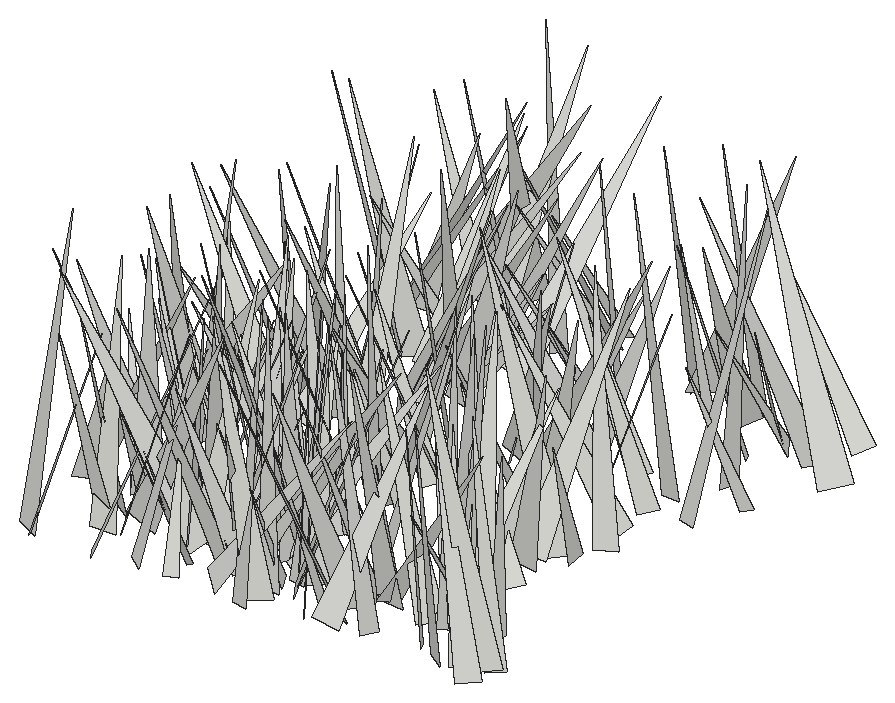
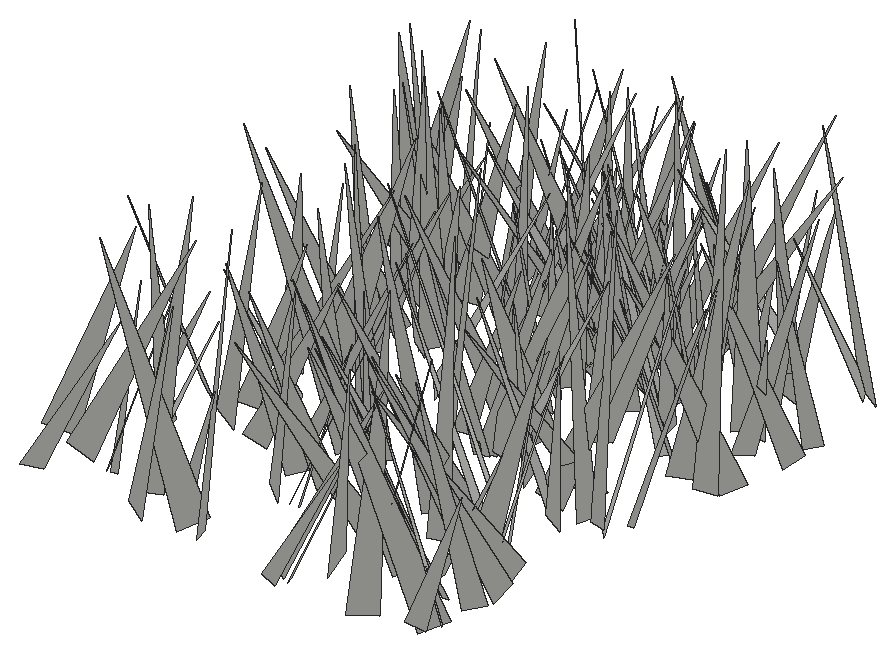
# SketchUp Ruby script. Lengths in inches.
U = 1.inch
M = Sketchup.active_model
def pt(a) = Geom::Point3d.new(a.map { |v| v * U })
def face(e, loops, mat)
  f = e.add_face(loops[0].map { |a| pt(a) })
  loops[1..].each { |l| e.add_face(l.map { |a| pt(a) }).erase! }
  f.material = f.back_material = mat if mat
  f
end
# faces: each face lists its corners as indices into pts; further lists are holes
def faces(e, pts, list, mat = nil) = list.each { |f| face(e, (f[0].is_a?(Array) ? f : [f]).map { |l| l.map { |i| pts[i] } }, mat) }
# xy, xz, yz: faces in a plane at the given z, y or x. An outline is a flat list of corners, or four numbers for a rectangle; further outlines are holes
def ring(l) = l.size == 4 ? [[l[0], l[1]], [l[2], l[1]], [l[2], l[3]], [l[0], l[3]]] : l.each_slice(2).to_a
def flat(e, list, mat, &to3) = list.each { |f| face(e, (f[0].is_a?(Array) ? f : [f]).map { |l| ring(l).map { |u, v| to3.(u, v) } }, mat) }
def xy(e, z, list, mat = nil) = flat(e, list, mat) { |x, y| [x, y, z] }
def xz(e, y, list, mat = nil) = flat(e, list, mat) { |x, z| [x, y, z] }
def yz(e, x, list, mat = nil) = flat(e, list, mat) { |y, z| [x, y, z] }
def lines(e, pts, list) = list.each { |a, b| e.add_line(pt(pts[a]), pt(pts[b])) }
# prism: a flat outline (further loops are holes) pulled along v
def prism(e, loops, v, mat = nil)
  f = face(e, loops, mat); d = Geom::Vector3d.new(v.map { |x| x * U })
  f.pushpull(f.normal.samedirection?(d) ? d.length : -d.length)
end
def box(e, o, s, mat = nil) = prism(e, [[o, [o[0] + s[0], o[1], o[2]], [o[0] + s[0], o[1] + s[1], o[2]], [o[0], o[1] + s[1], o[2]]]], [0, 0, s[2]], mat)
def at(x, y, z, deg = 0) = Geom::Transformation.translation(pt([x, y, z])) * Geom::Transformation.rotation(ORIGIN, Z_AXIS, deg.degrees)
def axes(o, x, y, z) = Geom::Transformation.new([*x, 0, *y, 0, *z, 0, *pt(o).to_a, 1])
def part(name) = M.definitions.add(name)
# library, detail: a bought-in or finely detailed component or shape, given as its bounding box
def library(name, o, s) = part(name).tap { |d| box(d.entities, o, s) }
def detail(e, o, s) = box(e.add_group.entities, o, s)
def put(e, d, t, mat = nil) = e.add_instance(d, t).tap { |i| i.material = mat if mat }
def group(e, t, mat = nil) = e.add_group.tap { |g| g.transformation = t; g.material = mat if mat }.entities
root = M.entities
c1 = part("fur_instance\#9")
p = [[0.8125,0,1.79],[0.67,-0.02,1.48],[0,-0.11,0],[0,0.11,0]]
faces(c1.entities,p,[[0,1,2,3]])
put(root,c1,axes([495.38,140.03,-21.86],[-4.54236,-5.48641,0.31776],[-5.31376,4.27953,-2.06985],[-1.40202,1.55551,6.81539]))
put(root,c1,axes([478.11,137.65,-21.86],[3.67219,7.15908,2.03524],[7.27938,-3.92759,0.68132],[-1.55086,-1.48365,8.01705]))
put(root,c1,axes([486.375,138.22,-21.86],[-1.12302,3.48075,0.37457],[3.50037,1.10997,0.18007],[-0.0574,-0.41163,3.65299]))
put(root,c1,axes([491.2,138.83,-21.66],[-2.35431,6.5098,1.98677],[6.74258,1.94391,1.62058],[-0.92858,-2.38982,6.73008]))
put(root,c1,axes([478.44,137.5,-21.86],[4.4489,2.71988,0.66857],[2.4928,-4.41728,1.38241],[-1.27698,0.85286,5.02786]))
put(root,c1,axes([480.96,140.17,-21.86],[-1.01611,-5.1437,1.43202],[-5.3112,0.8243,-0.80778],[-0.54728,1.55038,5.1805]))
put(root,c1,axes([495.01,141.31,-21.86],[2.20766,-6.15742,1.48059],[-5.96151,-2.54967,-1.71445],[-2.13691,0.75174,6.31254]))
put(root,c1,axes([501.15,139.78,-21.86],[3.12486,4.78234,3.10342],[5.39282,-3.6275,0.15986],[-1.8492,-2.49745,5.71052]))
put(root,c1,axes([484.2,138.2,-21.86],[3.27247,4.57721,0.86039],[4.6176,-3.3258,0.13012],[-0.60735,-0.62316,5.62521]))
put(root,c1,axes([485.58,141.44,-21.86],[-7.87957,1.88276,1.17896],[2.17634,7.41366,2.70618],[0.44527,-2.91806,7.63603]))
put(root,c1,axes([488.63,140.88,-21.86],[-4.94323,1.53486,1.76986],[2.06825,4.80019,1.61379],[1.10026,-2.12747,4.91803]))
put(root,c1,axes([490.85,141.14,-21.86],[-3.02452,-1.82217,1.01563],[-1.34667,3.07159,1.50047],[1.5932,-0.86291,3.19635]))
put(root,c1,axes([488.09,139.11,-21.86],[4.06376,5.39951,0.02576],[4.83357,-3.62337,-3.0294],[2.40665,-1.8401,6.04083]))
put(root,c1,axes([488.09,140.34,-21.66],[-2.1287,-6.56011,1.58213],[-6.38568,1.42177,-2.69649],[-2.18201,2.23898,6.34786]))
put(root,c1,axes([487.89,141.95,-21.86],[4.75134,-2.11282,0.36953],[-1.90852,-4.57438,-1.61505],[-0.97883,-1.33672,4.94275]))
put(root,c1,axes([482.17,141.16,-21.66],[1.4912,-7.63112,1.5604],[-7.07021,-0.65953,3.53123],[3.26816,2.05513,6.92734]))
put(root,c1,axes([494.4,139.97,-21.86],[0.25275,3.74041,1.98428],[3.79537,-1.08135,1.55493],[-1.87703,-1.68284,3.41127]))
put(root,c1,axes([493.27,139.68,-21.86],[5.9616,4.7587,3.0284],[5.08757,-6.43918,0.10304],[-2.43578,-1.80245,7.62727]))
put(root,c1,axes([490.82,137.81,-21.66],[3.07038,6.62387,1.59445],[6.28566,-3.42873,2.13997],[-2.62838,-0.46188,6.98022]))
put(root,c1,axes([486.28,139.74,-21.86],[-5.6206,-6.05261,0.8091],[-5.56666,4.62654,-4.06048],[-2.5102,3.29256,7.1929]))
put(root,c1,axes([503.71,139.0625,-21.86],[-1.94953,6.2532,0.70862],[6.08536,1.68405,1.8809],[-1.60411,-1.2111,6.27419]))
put(root,c1,axes([490.73,140.1,-21.86],[1.00735,6.64791,2.58508],[7.07427,-1.26504,0.49655],[-0.91221,-2.46923,6.70544]))
put(root,c1,axes([480.6,141.73,-21.86],[-3.05463,-4.97038,1.37571],[-5.09206,3.16016,0.11108],[0.81742,1.11209,5.83293]))
put(root,c1,axes([487.41,141.22,-21.66],[6.19787,3.91116,1.13836],[4.069,-5.84754,-2.06304],[0.19042,-2.34857,7.0324]))
put(root,c1,axes([488.89,141.14,-21.86],[3.67258,4.04026,0.63824],[3.75616,-2.99162,-2.6759],[1.61937,-2.22383,4.75932]))
put(root,c1,axes([503.95,140.1875,-21.66],[-2.60972,7.0339,1.93347],[7.14895,2.0575,2.16424],[-1.45142,-2.51309,7.18348]))
put(root,c1,axes([482.04,137.59,-21.86],[6.02604,4.35688,0.13616],[4.14402,-5.7981,2.12678],[-1.35204,1.64734,7.12547]))
put(root,c1,axes([495.26,142.71,-21.86],[-5.52274,-3.05851,1.02558],[-2.84433,5.57616,1.31266],[1.52186,-0.67738,6.17511]))
put(root,c1,axes([481.02,139.73,-21.86],[-0.28002,6.79198,1.74012],[7.00527,0.19856,0.35229],[-0.29175,-1.75129,6.78861]))
put(root,c1,axes([491.78,140.8125,-21.86],[4.36053,2.62617,0.62372],[2.69593,-4.29581,-0.7602],[-0.13318,-0.97427,5.03319]))
put(root,c1,axes([481.64,140.51,-21.86],[5.1332,2.66859,0.80867],[2.72409,-5.16107,-0.26035],[-0.59552,-0.60587,5.77956]))
put(root,c1,axes([481.54,142.61,-21.86],[2.09335,-3.21544,0.11512],[-3.16402,-2.08217,-0.6229],[-0.58423,-0.24481,3.78592]))
put(root,c1,axes([495.1,138.96,-21.66],[-1.51128,6.4389,0.97646],[6.11666,1.74753,-2.05657],[2.23592,-0.42848,6.28601]))
put(root,c1,axes([500.01,140.15,-21.66],[-4.46035,-2.40279,1.6408],[-2.85913,4.17643,-1.65628],[0.53948,2.26814,4.788]))
put(root,c1,axes([496.14,142.61,-21.86],[-0.46017,-7.01963,1.64197],[-7.20868,0.46604,-0.02793],[0.07879,1.64032,7.03464]))
put(root,c1,axes([502.37,142.23,-21.86],[-1.30366,-3.70433,0.26528],[-3.50778,1.13584,-1.37745],[-1.21983,0.69265,3.67753]))
put(root,c1,axes([502.68,139.71,-21.66],[-0.8171,5.77252,0.59098],[5.63961,0.64951,1.4532],[-1.36602,-0.77139,5.64605]))
put(root,c1,axes([497.35,139.51,-21.66],[-7.36083,-0.13148,0.37404],[-0.23398,7.05478,-2.12469],[0.32007,2.13349,7.04874]))
put(root,c1,axes([490.09,143.64,-21.66],[-5.41835,-3.58553,1.38238],[-3.2455,5.54933,1.6725],[2.0576,-0.68883,6.27832]))
put(root,c1,axes([504.11,140.64,-21.86],[-0.60049,6.11637,0.8715],[5.86899,0.29123,2.00004],[-1.92986,-1.0175,5.81123]))
put(root,c1,axes([486.98,141.81,-21.86],[4.2362,2.18763,0.04516],[2.18011,-4.21144,-0.49393],[0.18673,-0.4595,4.74206]))
put(root,c1,axes([485.09,141.32,-21.86],[-5.05417,-1.27819,2.14403],[-1.86511,5.15169,-1.32541],[1.65892,1.89778,5.04199]))
put(root,c1,axes([489.8,143.27,-21.86],[6.10585,-2.9623,2.45846],[-2.96929,-6.55789,-0.52733],[-2.45002,0.56525,6.76598]))
put(root,c1,axes([487.97,143.39,-21.66],[4.31656,-7.06636,0.27005],[-6.24466,-3.6606,4.0303],[3.31821,2.3034,7.23345]))
put(root,c1,axes([496.09,142.49,-21.66],[4.90095,-2.69617,0.00541],[-2.57457,-4.67657,1.67032],[0.80058,1.46597,5.33842]))
put(root,c1,axes([498.76,142.41,-21.86],[-3.37701,5.49526,1.43426],[5.6473,3.0721,1.52623],[-0.60248,-2.00587,6.26679]))
put(root,c1,axes([477.0625,143.12,-21.86],[3.32524,-3.2763,0.88677],[-3.39381,-3.22791,0.80025],[-0.05063,1.1934,4.59902]))
put(root,c1,axes([490.45,142.85,-21.86],[-3.74017,-2.83655,2.38458],[-3.12746,4.23356,0.13062],[1.98777,1.32365,4.69232]))
put(root,c1,axes([490.13,143.49,-21.86],[-0.66847,-3.61729,0.84651],[-3.58891,0.40659,-1.09666],[-0.95975,0.99906,3.51127]))
put(root,c1,axes([480.5,143.78,-21.86],[5.05478,-5.09898,2.04992],[-5.28407,-5.27475,-0.09077],[-1.51011,1.38923,7.17929]))
put(root,c1,axes([502.18,143.11,-21.86],[-4.58199,0.67037,2.42399],[0.81188,5.16228,0.10702],[2.38033,-0.47034,4.62953]))
put(root,c1,axes([484.65,143.41,-21.86],[7.55648,0.00384,2.83421],[0.13477,-8.06186,-0.34839],[-2.831,-0.37353,7.54844]))
put(root,c1,axes([495.88,143.53,-21.86],[-3.08604,-1.58363,1.00431],[-1.62158,3.22493,0.10239],[0.94181,0.36349,3.46714]))
put(root,c1,axes([489.42,144.56,-21.66],[-2.75065,-6.97463,1.22589],[-6.99898,2.47729,-1.60986],[-1.07823,1.71227,7.32256]))
put(root,c1,axes([486.96,143.85,-21.86],[-1.35927,-4.19334,1.10265],[-4.18909,0.97193,-1.4678],[-1.11869,1.45561,4.1566]))
put(root,c1,axes([500.625,142.46,-21.86],[2.96295,7.07925,2.39249],[7.30087,-3.29107,0.69644],[-1.59283,-1.91622,7.64263]))
put(root,c1,axes([499.76,142.66,-21.86],[-1.2405,4.10694,0.41743],[4.03089,1.11105,1.04764],[-0.89058,-0.69186,4.16031]))
put(root,c1,axes([484.1875,143.45,-21.86],[-6.45817,-1.9042,0.82118],[-2.02073,6.38203,-1.093],[0.4658,1.28531,6.64374]))
put(root,c1,axes([494.11,144.84,-21.66],[-5.74525,-5.95088,0.61636],[-5.93253,5.55629,-1.65334],[-0.77329,1.58601,8.10478]))
put(root,c1,axes([492.23,141.95,-21.86],[-5.70534,2.42628,0.74712],[2.22137,5.6608,-1.42016],[1.22905,1.03174,6.03498]))
put(root,c1,axes([491.39,141.46,-21.86],[2.9038,6.51052,1.10748],[6.2299,-3.10193,1.9005],[-2.1913,-0.1914,6.87074]))
put(root,c1,axes([485.47,141.67,-21.86],[-5.22484,3.83291,1.4033],[3.4058,5.3502,-1.93269],[2.24967,0.80218,6.18505]))
put(root,c1,axes([490.49,143.14,-21.86],[-2.02202,5.92033,1.45384],[6.05855,1.78151,1.17164],[-0.67672,-1.74024,6.14542]))
put(root,c1,axes([486.75,145,-21.86],[-5.73221,-5.07274,1.73381],[-5.23258,5.8463,-0.19467],[1.1657,1.29813,7.652]))
put(root,c1,axes([490.45,144.02,-21.86],[2.1369,3.02619,1.55246],[3.28055,-2.31782,0.00255],[-0.89775,-1.26656,3.70461]))
put(root,c1,axes([501.42,142.41,-21.86],[-5.51425,5.90533,1.65371],[5.90522,5.71303,-0.71018],[1.6541,-0.70927,8.04832]))
put(root,c1,axes([491.57,141.53,-21.86],[5.91646,3.40669,0.5347],[3.12979,-5.75065,2.00759],[-1.44773,1.49011,6.52531]))
put(root,c1,axes([489.68,144.2,-21.66],[-3.57331,4.48467,0.98446],[4.4978,3.16833,1.89248],[-0.92266,-1.92337,5.41289]))
put(root,c1,axes([478.97,146.0625,-21.66],[5.01755,-2.86523,2.69296],[-2.1597,-5.65647,-1.99435],[-3.28592,-0.6574,5.42291]))
put(root,c1,axes([489.03,141.4,-21.86],[-7.37463,3.18086,0.67882],[2.84062,7.11825,-2.49505],[1.58417,2.04365,7.63399]))
put(root,c1,axes([485.59,142.85,-21.86],[0.65103,4.23875,0.31259],[3.78552,-0.72206,1.9071],[-1.9325,0.01355,3.84107]))
put(root,c1,axes([499.49,143.52,-21.86],[-5.34624,-2.21651,3.3319],[-3.00843,5.89263,-0.90721],[2.6389,2.22728,5.71596]))
put(root,c1,axes([489.46,142.97,-21.86],[2.23337,6.49328,0.05356],[5.9184,-2.0122,-2.84202],[2.67172,-0.9705,6.25089]))
put(root,c1,axes([494.8,142.93,-21.86],[4.44163,5.80553,0.93246],[5.82565,-4.50337,0.28854],[-0.79717,-0.56325,7.30404]))
put(root,c1,axes([484.78,144.73,-21.86],[4.81991,2.46867,0.79438],[2.57067,-4.76928,-0.77622],[-0.3421,-1.05666,5.35942]))
put(root,c1,axes([482.05,145.16,-21.86],[-4.92159,1.07561,1.43405],[1.22896,5.07505,0.41117],[1.30503,-0.72281,5.02095]))
put(root,c1,axes([499.94,142.1875,-21.66],[-7.67594,0.43258,1.18162],[-0.05572,7.18028,-2.99063],[1.25708,2.9597,7.0826]))
put(root,c1,axes([483.38,143.76,-21.66],[-1.50811,5.89701,0.63499],[5.61901,1.21081,2.10069],[-1.89858,-1.1007,5.71281]))
put(root,c1,axes([499.87,142.15,-21.66],[-2.9172,5.75801,0.16061],[5.28877,2.74872,-2.48273],[2.2824,0.99014,5.95825]))
put(root,c1,axes([479.8,144.08,-21.86],[-1.23895,4.11427,0.01816],[3.97981,1.19363,1.09497],[-1.04341,-0.33255,4.15491]))
put(root,c1,axes([476.86,144.88,-21.86],[5.89255,-1.31891,0.46121],[-1.38894,-5.74659,1.31223],[-0.15186,1.38261,5.89404]))
put(root,c1,axes([487.06,147.18,-21.66],[-5.99784,0.36822,0.31916],[0.44096,5.77868,1.61988],[0.20737,-1.63795,5.78668]))
put(root,c1,axes([483.6,143.47,-21.86],[4.67368,1.9817,0.84614],[1.46066,-4.3994,2.23565],[-1.58416,1.79011,4.55767]))
put(root,c1,axes([484.43,145.33,-21.86],[-3.14834,2.92622,0.07201],[2.87738,3.07451,0.86494],[-0.53726,-0.68166,4.21031]))
put(root,c1,axes([500.14,144.29,-21.66],[0.70044,7.59304,1.85976],[7.56257,-1.13109,1.76971],[-1.98005,-1.63401,7.41708]))
put(root,c1,axes([497.0625,146.8,-21.86],[6.65936,-3.07974,1.86174],[-3.09449,-6.89952,-0.34452],[-1.83712,0.458,7.32893]))
put(root,c1,axes([489.75,145.78,-21.86],[-5.4066,3.91291,1.98693],[4.14231,5.59139,0.26032],[1.44915,-1.38406,6.66892]))
put(root,c1,axes([489.8125,144.11,-21.86],[-1.13883,5.42731,0.08742],[5.42427,1.13458,0.2244],[-0.2017,-0.13157,5.54096]))
put(root,c1,axes([492.57,146.1,-21.86],[-3.60643,-6.53276,3.39182],[-7.2869,3.70246,-0.61691],[1.0404,3.28673,7.43658]))
put(root,c1,axes([484.5,145.45,-21.86],[1.86244,4.7215,0.55373],[4.68693,-1.72429,-1.06173],[0.79484,-0.89561,4.96326]))
put(root,c1,axes([486.22,145.92,-21.86],[-2.76968,5.79414,2.34049],[6.07448,3.09716,-0.47899],[1.46654,-1.88589,6.4042]))
put(root,c1,axes([481.88,148.47,-21.66],[6.81977,1.54998,0.06465],[1.44583,-6.24479,-2.79788],[0.56233,-2.74155,6.40965]))
put(root,c1,axes([489.875,146.77,-21.86],[2.36348,3.65871,1.87372],[3.9267,-2.64879,0.21906],[-1.21573,-1.4425,4.3502]))
put(root,c1,axes([479.78,149.6,-21.66],[5.20163,-5.29224,1.8402],[-4.95757,-5.51713,-1.85336],[-2.61089,-0.0677,7.18539]))
put(root,c1,axes([478.12,149.97,-21.66],[-1.25565,-8.18969,1.33935],[-8.04493,1.53362,1.83538],[2.03567,1.00923,8.07955]))
put(root,c1,axes([485.57,144.4,-21.86],[4.16098,5.56887,0.17793],[5.30628,-4.02846,1.99315],[-1.69922,1.05685,6.65984]))
put(root,c1,axes([490.02,146.58,-21.86],[1.64216,5.46326,1.64146],[5.44457,-2.0108,1.24565],[-1.70244,-1.16093,5.56707]))
put(root,c1,axes([488.74,148.52,-21.66],[3.06956,3.90435,1.71137],[4.25532,-2.68017,-1.51785],[0.25498,-2.27325,4.72887]))
put(root,c1,axes([499.9,147.3125,-21.66],[-3.00277,4.1066,0.06153],[3.92812,2.84936,1.52829],[-1.19912,-0.94951,4.85234]))
put(root,c1,axes([498.86,149.25,-21.66],[1.26894,-6.32164,1.3833],[-6.3592,-0.957,1.46001],[1.19887,1.6149,6.28026]))
put(root,c1,axes([487.07,146.75,-21.86],[-6.05277,2.56522,0.71834],[2.46544,6.06973,-0.90131],[1.00895,0.55714,6.51184]))
put(root,c1,axes([499.04,146.78,-21.66],[-3.77654,1.99621,0.89861],[1.50689,3.67022,-1.82025],[1.58796,1.26459,3.86442]))
put(root,c1,axes([477.2,148.97,-21.66],[3.63581,-6.29578,1.08718],[-5.74464,-2.67402,3.72648],[2.79605,2.69271,6.24254]))
put(root,c1,axes([483.26,146.54,-21.86],[-6.67208,0.88571,0.68005],[0.61302,6.34873,-2.25421],[0.93335,2.16166,6.3419]))
put(root,c1,axes([480.76,149.03,-21.66],[2.90459,3.11145,0.76807],[3.13189,-2.53582,-1.57117],[0.67994,-1.61126,3.9559]))
put(root,c1,axes([480.96,146.58,-21.86],[4.06044,6.49572,1.60929],[6.19974,-4.35997,1.95581],[-2.5194,-0.26008,7.4065]))
put(root,c1,axes([491.67,149.38,-21.66],[-1.39517,3.65073,1.37856],[3.73252,0.82124,1.60268],[-1.13865,-1.78115,3.56451]))
put(root,c1,axes([485.2,149.47,-21.66],[-7.15301,3.97515,0.71331],[4.02795,6.91641,1.848],[-0.2937,-1.95899,7.97197]))
put(root,c1,axes([497.26,147.67,-21.66],[1.37607,4.21587,0.41156],[3.82506,-1.42264,1.78368],[-1.81985,0.19763,4.06025]))
put(root,c1,axes([494.35,150.21,-21.66],[-5.23491,-4.53939,0.15815],[-4.43832,5.06084,-1.65066],[-0.96564,1.34804,6.72946]))
put(root,c1,axes([500.49,151.22,-21.66],[4.01864,-1.00258,0.99057],[-0.63294,-3.95809,-1.43832],[-1.25928,-1.21004,3.88405]))
put(root,c1,axes([498.57,151.16,-21.66],[-1.67937,-5.43767,0.87836],[-5.25266,1.30456,-1.96667],[-1.65811,1.37475,5.34049]))
put(root,c1,axes([488.53,153.57,-21.66],[5.3138,-2.81187,1.14067],[-1.98861,-4.96443,-2.9739],[-2.29198,-2.2118,5.22484]))
put(root,c1,axes([488.16,153.23,-21.66],[-0.28332,-7.79704,0.77926],[-7.68212,0.12267,-1.56569],[-1.54472,0.82004,7.64347]))
put(root,c1,axes([478.81,154.77,-21.66],[-5.2943,-3.28141,1.0592],[-2.29433,4.80125,3.40634],[2.57403,-2.46971,5.21479]))
put(root,c1,axes([488.83,150.91,-21.66],[-4.99082,4.3261,0.4502],[4.29852,4.80129,1.51542],[-0.66378,-1.43477,6.4286]))
put(root,c1,axes([499.73,150.95,-21.66],[-2.9065,7.574,1.65107],[7.44857,2.24028,2.83534],[-2.14716,-2.4809,7.60092]))
put(root,c1,axes([490.68,152.61,-21.66],[-3.29735,3.76242,1.32483],[3.9802,2.99017,1.41439],[-0.2628,-1.92005,4.79874]))
put(root,c1,axes([498.5625,150.2,-21.66],[-1.75958,6.89289,0.89816],[6.66639,1.93582,-1.79628],[1.96924,-0.39424,6.88342]))
put(root,c1,axes([490.35,149.93,-21.66],[7.12647,2.20024,1.82821],[1.44023,-6.99989,2.8102],[-2.47167,2.26505,6.90872]))
put(root,c1,axes([500.64,154.51,-21.66],[-6.49837,1.01991,0.13564],[1.01971,6.26851,1.71854],[-0.13717,-1.71841,6.34946]))
put(root,c1,axes([483.36,155.25,-21.66],[0.24896,-7.3468,1.55373],[-6.97419,-0.80255,-2.67734],[-2.78393,1.35351,6.84612]))
put(root,c1,axes([479.39,156.12,-21.66],[-5.06426,-4.56399,0.84014],[-4.29824,5.08189,1.69768],[1.74956,-0.72593,6.60262]))
put(root,c1,axes([480.08,155.71,-21.66],[-3.33298,-6.74445,1.96036],[-6.484,3.7887,2.01069],[2.69971,0.77298,7.24938]))
put(root,c1,axes([489.04,156,-21.66],[-3.9717,-6.10655,1.7462],[-5.81347,4.32471,1.90107],[2.55787,0.34722,7.03209]))
put(root,c1,axes([488.62,153.8125,-21.66],[-0.11529,-4.79427,2.44231],[-5.06003,0.9271,1.58106],[1.8292,2.26244,4.52754]))
put(root,c1,axes([480.81,155.58,-21.66],[7.66875,0.29762,1.40281],[0.64374,-7.5341,-1.92071],[-1.28143,-2.00373,7.43029]))
put(root,c1,axes([501.05,152.77,-21.66],[-0.8728,6.82324,1.17968],[6.78553,0.6058,1.51645],[-1.38016,-1.33658,6.7096]))
put(root,c1,axes([486.65,154.68,-21.66],[-5.69424,-4.56861,0.52497],[-4.47673,5.31586,-2.29625],[-1.05201,2.10752,6.92992]))
put(root,c1,axes([493.01,157.19,-21.66],[-1.64763,-7.14584,1.34901],[-6.49832,2.06763,3.01567],[3.26416,0.50931,6.68457]))
put(root,c1,axes([487.23,151.05,-21.66],[-7.03666,4.34174,0.35439],[3.96979,6.66848,-2.87454],[1.79361,2.2741,7.75256]))
put(root,c1,axes([491.99,157.26,-21.66],[0.44147,-7.17503,0.62576],[-6.54369,-0.13768,3.03788],[3.00878,0.75334,6.51516]))
put(root,c1,axes([485.42,154.17,-21.66],[-5.55203,-0.57439,2.02149],[-1.15794,5.60149,-1.58866],[1.75372,1.88009,5.3508]))
put(root,c1,axes([494.51,156.91,-21.66],[1.53942,-5.44162,0.89342],[-5.38829,-1.28703,1.44538],[1.17292,1.22946,5.46735]))
put(root,c1,axes([493.77,157,-21.66],[6.6749,-4.96789,0.00129],[-4.8195,-6.47499,2.02019],[1.20515,1.62135,8.07174]))
put(root,c1,axes([482.04,153.47,-21.66],[-1.93127,6.17376,0.09606],[5.65668,1.80943,-2.5656],[2.47519,0.68189,5.93825]))
put(root,c1,axes([500.32,156.92,-21.66],[-2.9134,4.03937,1.46912],[4.26943,2.51447,1.5531],[-0.49677,-2.07934,4.73205]))
put(root,c1,axes([484.7,157.44,-21.66],[7.11507,4.33314,0.48127],[4.20256,-6.57141,-2.9643],[1.16029,-2.76992,7.78545]))
put(root,c1,axes([498.41,155.23,-21.66],[4.22042,3.02936,0.44277],[2.70703,-4.0447,1.87014],[-1.43005,1.2839,4.84681]))
put(root,c1,axes([495.32,159.22,-21.66],[-6.50951,0.22142,0.60358],[0.38251,6.26967,1.82536],[0.51674,-1.85181,6.25226]))
put(root,c1,axes([483.3,155.34,-21.66],[5.52585,4.05046,1.31825],[3.69086,-5.63091,1.83015],[-2.12639,0.75214,6.60241]))
put(root,c1,axes([481.89,156.82,-21.66],[1.02305,5.31057,1.33507],[5.15193,-1.39366,1.59576],[-1.8553,-0.94167,5.16743]))
put(root,c1,axes([484.66,158.64,-21.66],[6.0574,2.72005,0.2303],[2.69232,-5.86042,-1.5971],[0.45071,-1.54939,6.44516]))
put(root,c1,axes([486.82,159.52,-21.66],[1.53835,-7.01276,2.03333],[-7.04829,-0.88366,2.28484],[1.90652,2.39168,6.80623]))
put(root,c1,axes([481.24,161.21,-21.66],[-2.96228,-3.48582,0.87467],[-2.85625,2.97145,2.16874],[2.18125,-0.843,4.02773]))
put(root,c1,axes([500.28,158.63,-21.66],[1.97558,6.78512,3.04566],[6.89111,-2.85534,1.89119],[-2.79761,-2.24188,6.80913]))
put(root,c1,axes([492.22,156.54,-21.66],[4.15865,3.49208,0.81847],[2.77358,-3.92559,2.6563],[-2.27416,1.59814,4.73636]))
put(root,c1,axes([485.08,161.47,-21.66],[-0.53699,-7.34105,1.16615],[-7.27133,0.76139,1.44476],[1.5423,1.0337,7.21748]))
put(root,c1,axes([503.86,159.96,-21.66],[-0.24742,-3.68689,1.2628],[-3.55064,-0.30834,-1.59591],[-1.60648,1.24932,3.33279]))
put(root,c1,axes([497.86,159.44,-21.66],[-2.44299,5.49091,1.30941],[5.27932,1.71736,2.64808],[-1.99837,-2.17564,5.395]))
put(root,c1,axes([492.93,162.85,-21.66],[-4.66281,-2.88259,0.04543],[-2.761,4.48988,1.50703],[0.82963,-1.25893,5.27068]))
put(root,c1,axes([502.4,157.21,-21.66],[3.79972,6.90357,0.39781],[6.61789,-3.76205,2.07507],[-2.00527,0.66563,7.60206]))
put(root,c1,axes([484.875,159.77,-21.66],[6.3813,-2.25892,0.20905],[-2.20352,-6.02357,2.17449],[0.53935,2.11689,6.41056]))
put(root,c1,axes([492.47,160.6,-21.66],[3.58397,-3.64133,0.7361],[-3.60405,-3.15993,1.91614],[0.90107,1.84433,4.7363]))
put(root,c1,axes([492.23,163.07,-21.66],[-3.17214,-2.54983,0.51656],[-2.07776,2.97317,1.9168],[1.56569,-1.22048,3.59026]))
put(root,c1,axes([494.35,160.55,-21.66],[3.63193,-4.05591,1.60644],[-4.34601,-3.18259,1.79036],[0.37856,2.37544,5.14159]))
put(root,c1,axes([485.71,158.42,-21.66],[-4.47907,3.89554,0.463],[3.44419,4.24137,-2.36643],[1.87807,1.51235,5.44401]))
put(root,c1,axes([486.16,162.01,-21.66],[2.45066,3.05169,0.44917],[2.65928,-1.79957,-2.28257],[1.56295,-1.7231,3.17938]))
put(root,c1,axes([482.33,161.84,-21.66],[0.18988,-6.4583,3.19895],[-6.79344,-1.22898,-2.07794],[-2.40669,2.95955,6.11783]))
put(root,c1,axes([481.54,161.74,-21.66],[-6.3033,-3.29184,1.05702],[-3.45211,6.11366,-1.54635],[0.19083,1.86335,6.94094]))
put(root,c1,axes([485.68,162.27,-21.66],[2.51119,2.94201,0.30611],[2.79372,-2.22715,-1.51331],[0.97173,-1.19981,3.55969]))
put(root,c1,axes([482.82,164.2,-21.66],[-4.59731,-1.23154,0.33008],[-1.08177,4.4213,1.42926],[0.67485,-1.30242,4.53973]))
put(root,c1,axes([501.77,161.24,-21.66],[-7.13651,-0.0123,2.39844],[-0.61978,7.28244,-1.80677],[2.31701,1.91008,6.90402]))
put(root,c1,axes([494.06,162.75,-21.66],[-3.8782,-4.63911,2.52217],[-5.26639,3.62608,-1.42825],[0.38461,2.87286,5.87554]))
put(root,c1,axes([501.56,165.97,-21.66],[-3.93384,-2.91751,0.42121],[-2.51987,3.69278,2.04402],[1.52955,-1.41982,4.45073]))
put(root,c1,axes([498.68,166.47,-21.66],[5.9537,-4.05045,0.58701],[-3.75603,-5.81897,-2.05648],[-1.62572,-1.38951,6.90098]))
put(root,c1,axes([483.4,161.26,-21.66],[-1.05391,6.67902,0.37292],[6.52998,1.10912,-1.41007],[1.4518,-0.14015,6.613]))
put(root,c1,axes([501.14,165.9375,-21.66],[-2.16154,-4.08693,0.6496],[-3.73051,2.24163,1.68984],[1.79115,-0.26331,4.30345]))
put(root,c1,axes([500.71,163.9,-21.66],[-4.67684,-2.75,0.36196],[-2.71074,4.38122,-1.73872],[-0.58771,1.67594,5.13928]))
put(root,c1,axes([480.17,161.69,-21.66],[6.45135,0.1489,0.38361],[-0.04006,-5.77049,2.9136],[-0.40954,2.91007,5.75787]))
put(root,c1,axes([484.93,164.55,-21.66],[5.1253,5.35023,0.94765],[5.22805,-4.50107,-2.86349],[1.48003,-2.62814,6.83331]))
put(root,c1,axes([503.68,165.39,-21.66],[-2.36054,6.29762,2.85628],[6.53149,1.03928,3.10644],[-2.27111,-3.55673,5.96508]))
put(root,c1,axes([479.49,163.58,-21.66],[7.04502,0.38941,0.11832],[0.34745,-6.82295,1.76766],[-0.21195,1.75889,6.83077]))
put(root,c1,axes([479.64,165.55,-21.66],[3.48254,-4.50934,1.30252],[-4.66936,-3.1635,1.53235],[0.47726,1.95368,5.48763]))
put(root,c1,axes([505.78,164.32,-21.66],[-4.22364,6.9226,0.63988],[6.72709,3.88063,2.42031],[-1.75445,-1.78585,7.73974]))
put(root,c1,axes([485.99,165.11,-21.66],[-6.23091,-2.8217,1.23434],[-3.03851,6.08694,-1.42355],[0.50305,1.81577,6.69027]))
put(root,c1,axes([481.29,165.69,-21.66],[4.41498,5.25807,0.18984],[4.81628,-3.93899,-2.90917],[2.11822,-2.00311,6.21901]))
put(root,c1,axes([494.1875,168.1,-21.66],[-6.11732,-3.75265,2.76683],[-3.28898,6.70851,1.82699],[3.3046,-0.26993,6.94018]))
put(root,c1,axes([496.86,165.87,-21.66],[0.33091,4.05955,1.18914],[3.81261,-0.80293,1.68011],[-1.83248,-0.93747,3.71034]))
put(root,c1,axes([483.33,169.39,-21.66],[6.57894,-4.30915,0.69378],[-4.10201,-6.53322,-1.6802],[-1.49116,-1.03963,7.68298]))
put(root,c1,axes([488.18,168.92,-21.66],[-4.30266,-2.43803,0.04686],[-2.30354,4.09498,1.544],[0.79994,-1.32144,4.69819]))
put(root,c1,axes([487.06,163.4,-21.66],[-2.37553,7.32496,0.20013],[6.77476,2.27563,-2.87444],[2.79244,0.71043,7.14393]))
put(root,c1,axes([489.23,168.47,-21.66],[-2.79932,-5.24784,0.26282],[-5.09915,2.64134,-1.57068],[-1.26789,0.96362,5.73663]))
put(root,c1,axes([479.86,167.65,-21.66],[5.30447,3.34271,0.68413],[3.37643,-4.96043,-1.94241],[0.49141,-1.99988,5.96139]))
put(root,c1,axes([479.98,168.1875,-21.66],[3.5795,-7.50714,1.0436],[-6.77337,-2.6505,4.166],[3.40115,2.62237,7.19823]))
put(root,c1,axes([484.29,164.63,-21.66],[-4.73234,6.09922,1.47861],[5.53404,4.92888,-2.61961],[2.95993,0.53615,7.26177]))
put(root,c1,axes([504.56,167.94,-21.66],[-4.43376,3.47486,0.22998],[3.34427,4.14468,1.85019],[-0.97128,-1.59146,5.32068]))
put(root,c1,axes([495.09,167.5625,-21.66],[6.69732,-3.52244,1.21858],[-3.71872,-6.48437,1.69431],[-0.25228,2.07171,7.37503]))
put(root,c1,axes([489,169.49,-21.66],[-0.33006,-3.76044,0.39687],[-3.50265,0.15395,-1.45434],[-1.42474,0.49269,3.4835]))
put(root,c1,axes([487.36,166.35,-21.66],[-7.91635,-0.39433,1.24518],[-0.80795,7.48837,-2.76517],[1.02625,2.85367,7.42819]))
put(root,c1,axes([498.09,168.23,-21.66],[1.91991,5.69676,2.84026],[5.7974,-2.78995,1.67703],[-2.62873,-1.9923,5.77292]))
put(root,c1,axes([480.75,168.6875,-21.66],[-2.13288,4.47426,0.69403],[4.36785,1.83113,1.61826],[-1.19274,-1.2953,4.68502]))
